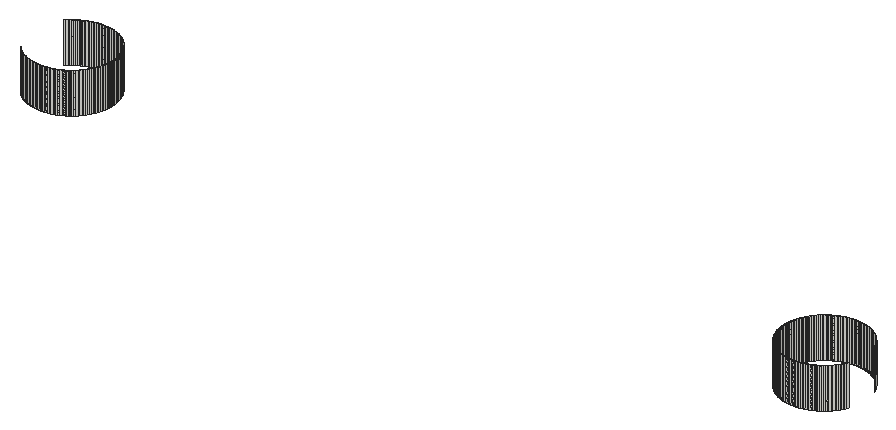
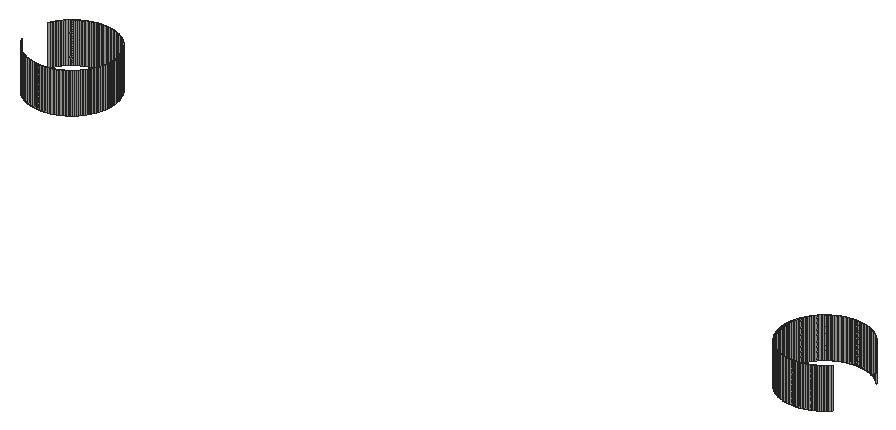
# SketchUp Ruby script. Lengths in inches.
U = 1.inch
M = Sketchup.active_model
def pt(a) = Geom::Point3d.new(a.map { |v| v * U })
def face(e, loops, mat)
  f = e.add_face(loops[0].map { |a| pt(a) })
  loops[1..].each { |l| e.add_face(l.map { |a| pt(a) }).erase! }
  f.material = f.back_material = mat if mat
  f
end
# faces: each face lists its corners as indices into pts; further lists are holes
def faces(e, pts, list, mat = nil) = list.each { |f| face(e, (f[0].is_a?(Array) ? f : [f]).map { |l| l.map { |i| pts[i] } }, mat) }
# xy, xz, yz: faces in a plane at the given z, y or x. An outline is a flat list of corners, or four numbers for a rectangle; further outlines are holes
def ring(l) = l.size == 4 ? [[l[0], l[1]], [l[2], l[1]], [l[2], l[3]], [l[0], l[3]]] : l.each_slice(2).to_a
def flat(e, list, mat, &to3) = list.each { |f| face(e, (f[0].is_a?(Array) ? f : [f]).map { |l| ring(l).map { |u, v| to3.(u, v) } }, mat) }
def xy(e, z, list, mat = nil) = flat(e, list, mat) { |x, y| [x, y, z] }
def xz(e, y, list, mat = nil) = flat(e, list, mat) { |x, z| [x, y, z] }
def yz(e, x, list, mat = nil) = flat(e, list, mat) { |y, z| [x, y, z] }
def lines(e, pts, list) = list.each { |a, b| e.add_line(pt(pts[a]), pt(pts[b])) }
# prism: a flat outline (further loops are holes) pulled along v
def prism(e, loops, v, mat = nil)
  f = face(e, loops, mat); d = Geom::Vector3d.new(v.map { |x| x * U })
  f.pushpull(f.normal.samedirection?(d) ? d.length : -d.length)
end
def box(e, o, s, mat = nil) = prism(e, [[o, [o[0] + s[0], o[1], o[2]], [o[0] + s[0], o[1] + s[1], o[2]], [o[0], o[1] + s[1], o[2]]]], [0, 0, s[2]], mat)
def at(x, y, z, deg = 0) = Geom::Transformation.translation(pt([x, y, z])) * Geom::Transformation.rotation(ORIGIN, Z_AXIS, deg.degrees)
def axes(o, x, y, z) = Geom::Transformation.new([*x, 0, *y, 0, *z, 0, *pt(o).to_a, 1])
def part(name) = M.definitions.add(name)
# library, detail: a bought-in or finely detailed component or shape, given as its bounding box
def library(name, o, s) = part(name).tap { |d| box(d.entities, o, s) }
def detail(e, o, s) = box(e.add_group.entities, o, s)
def put(e, d, t, mat = nil) = e.add_instance(d, t).tap { |i| i.material = mat if mat }
def group(e, t, mat = nil) = e.add_group.tap { |g| g.transformation = t; g.material = mat if mat }.entities
root = M.entities
xz(root,254,[[296.84,228,296.92,231],[296.92,228,297,231],[297,228,297.08,231],[297.08,228,297.16,231],[352.84,228,352.92,231],
  [352.92,228,353,231],[353,228,353.08,231],[353.08,228,353.16,231]])
xz(root,260,[[296.84,228,296.92,231],[296.92,228,297,231],[297,228,297.08,231],[297.08,228,297.16,231],[352.84,228,352.92,231],
  [352.92,228,353,231],[353,228,353.08,231],[353.08,228,353.16,231]])
yz(root,300,[[256.84,228,256.92,231],[256.92,228,257,231],[257,228,257.08,231],[257.08,228,257.16,231]])
yz(root,350,[[256.84,228,256.92,231],[256.92,228,257,231],[257,228,257.08,231],[257.08,228,257.16,231]])
p = [[296.53,254.04,228],[296.45,254.05,228],[296.45,254.05,231],[296.53,254.04,231],[296.61,254.03,228],[296.61,254.03,231],
  [296.6875,254.02,228],[296.6875,254.02,231],[296.76,254.01,228],[296.76,254.01,231],[296.84,254,228],[296.84,254,231],
  [297.24,254.01,228],[297.16,254,228],[297.16,254,231],[297.24,254.01,231],[297.3125,254.02,228],[297.3125,254.02,231],
  [297.39,254.03,228],[297.39,254.03,231],[297.47,254.04,228],[297.47,254.04,231],[297.55,254.05,228],[297.55,254.05,231],
  [352.53,254.04,228],[352.45,254.05,228],[352.45,254.05,231],[352.53,254.04,231],[352.61,254.03,228],[352.61,254.03,231],
  [352.6875,254.02,228],[352.6875,254.02,231],[352.76,254.01,228],[352.76,254.01,231],[352.84,254,228],[352.84,254,231],
  [353.24,254.01,228],[353.16,254,228],[353.16,254,231],[353.24,254.01,231],[353.3125,254.02,228],[353.3125,254.02,231],
  [353.39,254.03,228],[353.39,254.03,231],[353.47,254.04,228],[353.47,254.04,231],[353.55,254.05,228],[353.55,254.05,231],
  [296.07,254.15,228],[296,254.17,228],[296,254.17,231],[296.07,254.15,231],[296.15,254.125,228],[296.15,254.125,231],
  [296.22,254.1,228],[296.22,254.1,231],[296.3,254.08,228],[296.3,254.08,231],[296.375,254.07,228],[296.375,254.07,231],
  [297.625,254.07,228],[297.625,254.07,231],[297.7,254.08,228],[297.7,254.08,231],[297.78,254.1,228],[297.78,254.1,231],
  [297.85,254.125,228],[297.85,254.125,231],[297.93,254.15,228],[297.93,254.15,231],[298,254.17,228],[298,254.17,231],
  [352.07,254.15,228],[352,254.17,228],[352,254.17,231],[352.07,254.15,231],[352.15,254.125,228],[352.15,254.125,231],
  [352.22,254.1,228],[352.22,254.1,231],[352.3,254.08,228],[352.3,254.08,231],[352.375,254.07,228],[352.375,254.07,231],
  [353.625,254.07,228],[353.625,254.07,231],[353.7,254.08,228],[353.7,254.08,231],[353.78,254.1,228],[353.78,254.1,231],
  [353.85,254.125,228],[353.85,254.125,231],[353.93,254.15,228],[353.93,254.15,231],[354,254.17,228],[354,254.17,231],
  [295.85,254.23,228],[295.78,254.26,228],[295.78,254.26,231],[295.85,254.23,231],[295.92,254.2,228],[295.92,254.2,231],
  [298.08,254.2,228],[298.08,254.2,231],[298.15,254.23,228],[298.15,254.23,231],[298.22,254.26,228],[298.22,254.26,231],
  [351.85,254.23,228],[351.78,254.26,228],[351.78,254.26,231],[351.85,254.23,231],[351.92,254.2,228],[351.92,254.2,231],
  [354.08,254.2,228],[354.08,254.2,231],[354.15,254.23,228],[354.15,254.23,231],[354.22,254.26,228],[354.22,254.26,231],
  [295.64,254.33,228],[295.57,254.36,228],[295.57,254.36,231],[295.64,254.33,231],[295.71,254.29,228],[295.71,254.29,231],
  [298.29,254.29,228],[298.29,254.29,231],[298.36,254.33,228],[298.36,254.33,231],[298.43,254.36,228],[298.43,254.36,231],
  [351.64,254.33,228],[351.57,254.36,228],[351.57,254.36,231],[351.64,254.33,231],[351.71,254.29,228],[351.71,254.29,231],
  [354.29,254.29,228],[354.29,254.29,231],[354.36,254.33,228],[354.36,254.33,231],[354.43,254.36,228],[354.43,254.36,231],
  [295.43,254.44,228],[295.37,254.48,228],[295.37,254.48,231],[295.43,254.44,231],[295.5,254.4,228],[295.5,254.4,231],
  [298.5,254.4,228],[298.5,254.4,231],[298.57,254.44,228],[298.57,254.44,231],[298.63,254.48,228],[298.63,254.48,231],
  [351.43,254.44,228],[351.37,254.48,228],[351.37,254.48,231],[351.43,254.44,231],[351.5,254.4,228],[351.5,254.4,231],
  [354.5,254.4,228],[354.5,254.4,231],[354.57,254.44,228],[354.57,254.44,231],[354.63,254.48,228],[354.63,254.48,231],
  [295.3,254.53,228],[295.24,254.57,228],[295.24,254.57,231],[295.3,254.53,231],[298.7,254.53,228],[298.7,254.53,231],
  [298.76,254.57,228],[298.76,254.57,231],[351.3,254.53,228],[351.24,254.57,228],[351.24,254.57,231],[351.3,254.53,231],
  [354.7,254.53,228],[354.7,254.53,231],[354.76,254.57,228],[354.76,254.57,231],[295.17,254.62,228],[295.11,254.67,228],
  [295.11,254.67,231],[295.17,254.62,231],[298.83,254.62,228],[298.83,254.62,231],[298.89,254.67,228],[298.89,254.67,231],
  [351.17,254.62,228],[351.11,254.67,228],[351.11,254.67,231],[351.17,254.62,231],[354.83,254.62,228],[354.83,254.62,231],
  [354.89,254.67,228],[354.89,254.67,231],[295.05,254.72,228],[294.99,254.77,228],[294.99,254.77,231],[295.05,254.72,231],
  [298.95,254.72,228],[298.95,254.72,231],[299.01,254.77,228],[299.01,254.77,231],[351.05,254.72,228],[350.99,254.77,228],
  [350.99,254.77,231],[351.05,254.72,231],[354.95,254.72,228],[354.95,254.72,231],[355.01,254.77,228],[355.01,254.77,231],
  [294.93,254.82,228],[294.88,254.88,228],[294.88,254.88,231],[294.93,254.82,231],[299.07,254.82,228],[299.07,254.82,231],
  [299.12,254.88,228],[299.12,254.88,231],[350.93,254.82,228],[350.88,254.88,228],[350.88,254.88,231],[350.93,254.82,231],
  [355.07,254.82,228],[355.07,254.82,231],[355.12,254.88,228],[355.12,254.88,231],[294.82,254.93,228],[294.77,254.99,228],
  [294.77,254.99,231],[294.82,254.93,231],[299.18,254.93,228],[299.18,254.93,231],[299.23,254.99,228],[299.23,254.99,231],
  [350.82,254.93,228],[350.77,254.99,228],[350.77,254.99,231],[350.82,254.93,231],[355.18,254.93,228],[355.18,254.93,231],
  [355.23,254.99,228],[355.23,254.99,231],[299.28,255.05,228],[299.28,255.05,231],[350.72,255.05,228],[350.72,255.05,231],
  [355.28,255.05,228],[355.28,255.05,231],[299.33,255.11,228],[299.33,255.11,231],[299.38,255.17,228],[299.38,255.17,231],
  [350.67,255.11,228],[350.62,255.17,228],[350.62,255.17,231],[350.67,255.11,231],[355.33,255.11,228],[355.33,255.11,231],
  [355.38,255.17,228],[355.38,255.17,231],[299.43,255.24,228],[299.43,255.24,231],[299.47,255.3,228],[299.47,255.3,231],
  [350.57,255.24,228],[350.53,255.3,228],[350.53,255.3,231],[350.57,255.24,231],[355.43,255.24,228],[355.43,255.24,231],
  [355.47,255.3,228],[355.47,255.3,231],[299.52,255.37,228],[299.52,255.37,231],[350.48,255.37,228],[350.48,255.37,231],
  [355.52,255.37,228],[355.52,255.37,231],[299.56,255.43,228],[299.56,255.43,231],[299.6,255.5,228],[299.6,255.5,231],
  [350.44,255.43,228],[350.4,255.5,228],[350.4,255.5,231],[350.44,255.43,231],[355.56,255.43,228],[355.56,255.43,231],
  [355.6,255.5,228],[355.6,255.5,231],[299.64,255.57,228],[299.64,255.57,231],[350.36,255.57,228],[350.36,255.57,231],
  [355.64,255.57,228],[355.64,255.57,231],[299.67,255.64,228],[299.67,255.64,231],[299.71,255.71,228],[299.71,255.71,231],
  [350.33,255.64,228],[350.29,255.71,228],[350.29,255.71,231],[350.33,255.64,231],[355.67,255.64,228],[355.67,255.64,231],
  [355.71,255.71,228],[355.71,255.71,231],[299.74,255.78,228],[299.74,255.78,231],[350.26,255.78,228],[350.26,255.78,231],
  [355.74,255.78,228],[355.74,255.78,231],[299.77,255.85,228],[299.77,255.85,231],[350.23,255.85,228],[350.23,255.85,231],
  [299.8,255.92,228],[299.8,255.92,231],[299.83,256,228],[299.83,256,231],[350.2,255.92,228],[350.17,256,228],
  [350.17,256,231],[350.2,255.92,231],[299.85,256.07,228],[299.85,256.07,231],[350.15,256.07,228],[350.15,256.07,231],
  [299.875,256.15,228],[299.875,256.15,231],[299.9,256.22,228],[299.9,256.22,231],[350.125,256.15,228],[350.1,256.22,228],
  [350.1,256.22,231],[350.125,256.15,231],[299.92,256.3,228],[299.92,256.3,231],[350.08,256.3,228],[350.08,256.3,231],
  [299.93,256.375,228],[299.93,256.375,231],[350.07,256.375,228],[350.07,256.375,231],[299.95,256.45,228],[299.95,256.45,231],
  [350.05,256.45,228],[350.05,256.45,231],[299.96,256.53,228],[299.96,256.53,231],[299.97,256.61,228],[299.97,256.61,231],
  [350.04,256.53,228],[350.03,256.61,228],[350.03,256.61,231],[350.04,256.53,231],[299.98,256.6875,228],[299.98,256.6875,231],
  [350.02,256.6875,228],[350.02,256.6875,231],[299.99,256.76,228],[299.99,256.76,231],[350.01,256.76,228],[350.01,256.76,231],
  [300,256.84,228],[300,256.84,231],[350,256.84,228],[350,256.84,231],[299.98,257.3125,228],[299.99,257.24,228],
  [299.99,257.24,231],[299.98,257.3125,231],[300,257.16,228],[300,257.16,231],[350,257.16,228],[350.01,257.24,228],
  [350.01,257.24,231],[350,257.16,231],[350.02,257.3125,228],[350.02,257.3125,231],[299.97,257.39,228],[299.97,257.39,231],
  [350.03,257.39,228],[350.03,257.39,231],[299.96,257.47,228],[299.96,257.47,231],[350.04,257.47,228],[350.04,257.47,231],
  [299.93,257.625,228],[299.95,257.55,228],[299.95,257.55,231],[299.93,257.625,231],[350.05,257.55,228],[350.05,257.55,231],
  [350.07,257.625,228],[350.07,257.625,231],[299.92,257.7,228],[299.92,257.7,231],[350.08,257.7,228],[350.08,257.7,231],
  [299.9,257.78,228],[299.9,257.78,231],[350.1,257.78,228],[350.1,257.78,231],[299.875,257.85,228],[299.875,257.85,231],
  [350.125,257.85,228],[350.125,257.85,231],[299.83,258,228],[299.85,257.93,228],[299.85,257.93,231],[299.83,258,231],
  [350.15,257.93,228],[350.15,257.93,231],[350.17,258,228],[350.17,258,231],[299.8,258.08,228],[299.8,258.08,231],
  [350.2,258.08,228],[350.2,258.08,231],[299.74,258.22,228],[299.77,258.15,228],[299.77,258.15,231],[299.74,258.22,231],
  [350.23,258.15,228],[350.23,258.15,231],[350.26,258.22,228],[350.26,258.22,231],[299.71,258.29,228],[299.71,258.29,231],
  [350.29,258.29,228],[350.29,258.29,231],[355.71,258.29,228],[355.74,258.22,228],[355.74,258.22,231],[355.71,258.29,231],
  [299.67,258.36,228],[299.67,258.36,231],[350.33,258.36,228],[350.33,258.36,231],[355.67,258.36,228],[355.67,258.36,231],
  [299.6,258.5,228],[299.64,258.43,228],[299.64,258.43,231],[299.6,258.5,231],[350.36,258.43,228],[350.36,258.43,231],
  [350.4,258.5,228],[350.4,258.5,231],[355.6,258.5,228],[355.64,258.43,228],[355.64,258.43,231],[355.6,258.5,231],
  [299.56,258.57,228],[299.56,258.57,231],[350.44,258.57,228],[350.44,258.57,231],[355.56,258.57,228],[355.56,258.57,231],
  [299.47,258.7,228],[299.52,258.63,228],[299.52,258.63,231],[299.47,258.7,231],[350.48,258.63,228],[350.48,258.63,231],
  [350.53,258.7,228],[350.53,258.7,231],[355.47,258.7,228],[355.52,258.63,228],[355.52,258.63,231],[355.47,258.7,231],
  [299.43,258.76,228],[299.43,258.76,231],[350.57,258.76,228],[350.57,258.76,231],[355.43,258.76,228],[355.43,258.76,231],
  [299.33,258.89,228],[299.38,258.83,228],[299.38,258.83,231],[299.33,258.89,231],[350.62,258.83,228],[350.62,258.83,231],
  [350.67,258.89,228],[350.67,258.89,231],[355.33,258.89,228],[355.38,258.83,228],[355.38,258.83,231],[355.33,258.89,231],
  [299.23,259.01,228],[299.28,258.95,228],[299.28,258.95,231],[299.23,259.01,231],[350.72,258.95,228],[350.72,258.95,231],
  [350.77,259.01,228],[350.77,259.01,231],[355.23,259.01,228],[355.28,258.95,228],[355.28,258.95,231],[355.23,259.01,231],
  [294.77,259.01,228],[294.82,259.07,228],[294.82,259.07,231],[294.77,259.01,231],[299.18,259.07,228],[299.18,259.07,231],
  [350.82,259.07,228],[350.82,259.07,231],[355.18,259.07,228],[355.18,259.07,231],[294.88,259.12,228],[294.88,259.12,231],
  [294.93,259.18,228],[294.93,259.18,231],[299.07,259.18,228],[299.12,259.12,228],[299.12,259.12,231],[299.07,259.18,231],
  [350.88,259.12,228],[350.88,259.12,231],[350.93,259.18,228],[350.93,259.18,231],[355.07,259.18,228],[355.12,259.12,228],
  [355.12,259.12,231],[355.07,259.18,231],[294.99,259.23,228],[294.99,259.23,231],[295.05,259.28,228],[295.05,259.28,231],
  [298.95,259.28,228],[299.01,259.23,228],[299.01,259.23,231],[298.95,259.28,231],[350.99,259.23,228],[350.99,259.23,231],
  [351.05,259.28,228],[351.05,259.28,231],[354.95,259.28,228],[355.01,259.23,228],[355.01,259.23,231],[354.95,259.28,231],
  [295.11,259.33,228],[295.11,259.33,231],[295.17,259.38,228],[295.17,259.38,231],[298.83,259.38,228],[298.89,259.33,228],
  [298.89,259.33,231],[298.83,259.38,231],[351.11,259.33,228],[351.11,259.33,231],[351.17,259.38,228],[351.17,259.38,231],
  [354.83,259.38,228],[354.89,259.33,228],[354.89,259.33,231],[354.83,259.38,231],[295.24,259.43,228],[295.24,259.43,231],
  [295.3,259.47,228],[295.3,259.47,231],[298.7,259.47,228],[298.76,259.43,228],[298.76,259.43,231],[298.7,259.47,231],
  [351.24,259.43,228],[351.24,259.43,231],[351.3,259.47,228],[351.3,259.47,231],[354.7,259.47,228],[354.76,259.43,228],
  [354.76,259.43,231],[354.7,259.47,231],[295.37,259.52,228],[295.37,259.52,231],[295.43,259.56,228],[295.43,259.56,231],
  [298.57,259.56,228],[298.63,259.52,228],[298.63,259.52,231],[298.57,259.56,231],[351.37,259.52,228],[351.37,259.52,231],
  [351.43,259.56,228],[351.43,259.56,231],[354.57,259.56,228],[354.63,259.52,228],[354.63,259.52,231],[354.57,259.56,231],
  [295.5,259.6,228],[295.5,259.6,231],[295.57,259.64,228],[295.57,259.64,231],[295.64,259.67,228],[295.64,259.67,231],
  [298.36,259.67,228],[298.43,259.64,228],[298.43,259.64,231],[298.36,259.67,231],[298.5,259.6,228],[298.5,259.6,231],
  [351.5,259.6,228],[351.5,259.6,231],[351.57,259.64,228],[351.57,259.64,231],[351.64,259.67,228],[351.64,259.67,231],
  [354.36,259.67,228],[354.43,259.64,228],[354.43,259.64,231],[354.36,259.67,231],[354.5,259.6,228],[354.5,259.6,231],
  [295.71,259.71,228],[295.71,259.71,231],[295.78,259.74,228],[295.78,259.74,231],[295.85,259.77,228],[295.85,259.77,231],
  [298.15,259.77,228],[298.22,259.74,228],[298.22,259.74,231],[298.15,259.77,231],[298.29,259.71,228],[298.29,259.71,231],
  [351.71,259.71,228],[351.71,259.71,231],[351.78,259.74,228],[351.78,259.74,231],[351.85,259.77,228],[351.85,259.77,231],
  [354.15,259.77,228],[354.22,259.74,228],[354.22,259.74,231],[354.15,259.77,231],[354.29,259.71,228],[354.29,259.71,231],
  [295.92,259.8,228],[295.92,259.8,231],[296,259.83,228],[296,259.83,231],[296.07,259.85,228],[296.07,259.85,231],
  [297.93,259.85,228],[298,259.83,228],[298,259.83,231],[297.93,259.85,231],[298.08,259.8,228],[298.08,259.8,231],
  [351.92,259.8,228],[351.92,259.8,231],[352,259.83,228],[352,259.83,231],[352.07,259.85,228],[352.07,259.85,231],
  [353.93,259.85,228],[354,259.83,228],[354,259.83,231],[353.93,259.85,231],[354.08,259.8,228],[354.08,259.8,231],
  [296.15,259.875,228],[296.15,259.875,231],[296.22,259.9,228],[296.22,259.9,231],[296.3,259.92,228],[296.3,259.92,231],
  [296.375,259.93,228],[296.375,259.93,231],[296.45,259.95,228],[296.45,259.95,231],[296.53,259.96,228],[296.53,259.96,231],
  [297.47,259.96,228],[297.55,259.95,228],[297.55,259.95,231],[297.47,259.96,231],[297.625,259.93,228],[297.625,259.93,231],
  [297.7,259.92,228],[297.7,259.92,231],[297.78,259.9,228],[297.78,259.9,231],[297.85,259.875,228],[297.85,259.875,231],
  [352.15,259.875,228],[352.15,259.875,231],[352.22,259.9,228],[352.22,259.9,231],[352.3,259.92,228],[352.3,259.92,231],
  [352.375,259.93,228],[352.375,259.93,231],[352.45,259.95,228],[352.45,259.95,231],[352.53,259.96,228],[352.53,259.96,231],
  [353.47,259.96,228],[353.55,259.95,228],[353.55,259.95,231],[353.47,259.96,231],[353.625,259.93,228],[353.625,259.93,231],
  [353.7,259.92,228],[353.7,259.92,231],[353.78,259.9,228],[353.78,259.9,231],[353.85,259.875,228],[353.85,259.875,231],
  [296.61,259.97,228],[296.61,259.97,231],[296.6875,259.98,228],[296.6875,259.98,231],[296.76,259.99,228],[296.76,259.99,231],
  [296.84,260,228],[296.84,260,231],[297.16,260,228],[297.24,259.99,228],[297.24,259.99,231],[297.16,260,231],
  [297.3125,259.98,228],[297.3125,259.98,231],[297.39,259.97,228],[297.39,259.97,231],[352.61,259.97,228],[352.61,259.97,231],
  [352.6875,259.98,228],[352.6875,259.98,231],[352.76,259.99,228],[352.76,259.99,231],[352.84,260,228],[352.84,260,231],
  [353.16,260,228],[353.24,259.99,228],[353.24,259.99,231],[353.16,260,231],[353.3125,259.98,228],[353.3125,259.98,231],
  [353.39,259.97,228],[353.39,259.97,231]]
faces(root,p,[[0,1,2,3],[4,0,3,5],[6,4,5,7],[8,6,7,9],[10,8,9,11],[12,13,14,15],[16,12,15,17],[18,16,17,19],
  [20,18,19,21],[22,20,21,23],[24,25,26,27],[28,24,27,29],[30,28,29,31],[32,30,31,33],[34,32,33,35],[36,37,38,39],
  [40,36,39,41],[42,40,41,43],[44,42,43,45],[46,44,45,47],[48,49,50,51],[52,48,51,53],[54,52,53,55],[56,54,55,57],
  [58,56,57,59],[1,58,59,2],[60,22,23,61],[62,60,61,63],[64,62,63,65],[66,64,65,67],[68,66,67,69],[70,68,69,71],
  [72,73,74,75],[76,72,75,77],[78,76,77,79],[80,78,79,81],[82,80,81,83],[25,82,83,26],[84,46,47,85],[86,84,85,87],
  [88,86,87,89],[90,88,89,91],[92,90,91,93],[94,92,93,95],[96,97,98,99],[100,96,99,101],[49,100,101,50],[102,70,71,103],
  [104,102,103,105],[106,104,105,107],[108,109,110,111],[112,108,111,113],[73,112,113,74],[114,94,95,115],[116,114,115,117],[118,116,117,119],
  [120,121,122,123],[124,120,123,125],[97,124,125,98],[126,106,107,127],[128,126,127,129],[130,128,129,131],[132,133,134,135],[136,132,135,137],
  [109,136,137,110],[138,118,119,139],[140,138,139,141],[142,140,141,143],[144,145,146,147],[148,144,147,149],[121,148,149,122],[150,130,131,151],
  [152,150,151,153],[154,152,153,155],[156,157,158,159],[160,156,159,161],[133,160,161,134],[162,142,143,163],[164,162,163,165],[166,164,165,167],
  [168,169,170,171],[145,168,171,146],[172,154,155,173],[174,172,173,175],[176,177,178,179],[157,176,179,158],[180,166,167,181],[182,180,181,183],
  [184,185,186,187],[169,184,187,170],[188,174,175,189],[190,188,189,191],[192,193,194,195],[177,192,195,178],[196,182,183,197],[198,196,197,199],
  [200,201,202,203],[185,200,203,186],[204,190,191,205],[206,204,205,207],[208,209,210,211],[193,208,211,194],[212,198,199,213],[214,212,213,215],
  [216,217,218,219],[201,216,219,202],[220,206,207,221],[222,220,221,223],[224,225,226,227],[209,224,227,210],[228,214,215,229],[230,228,229,231],
  [232,233,234,235],[217,232,235,218],[236,222,223,237],[238,236,237,239],[240,241,242,243],[225,240,243,226],[244,230,231,245],[246,244,245,247],
  [248,238,239,249],[241,250,251,242],[252,246,247,253],[254,248,249,255],[256,254,255,257],[258,259,260,261],[250,258,261,251],[262,252,253,263],
  [264,262,263,265],[266,256,257,267],[268,266,267,269],[270,271,272,273],[259,270,273,260],[274,264,265,275],[276,274,275,277],[278,268,269,279],
  [271,280,281,272],[282,276,277,283],[284,278,279,285],[286,284,285,287],[288,289,290,291],[280,288,291,281],[292,282,283,293],[294,292,293,295],
  [296,286,287,297],[289,298,299,290],[300,294,295,301],[302,296,297,303],[304,302,303,305],[306,307,308,309],[298,306,309,299],[310,300,301,311],
  [312,310,311,313],[314,304,305,315],[307,316,317,308],[318,312,313,319],[320,314,315,321],[316,322,323,317],[324,320,321,325],[326,324,325,327],
  [328,329,330,331],[322,328,331,323],[332,326,327,333],[329,334,335,330],[336,332,333,337],[338,336,337,339],[340,341,342,343],[334,340,343,335],
  [344,338,339,345],[341,346,347,342],[348,344,345,349],[346,350,351,347],[352,348,349,353],[350,354,355,351],[356,352,353,357],[358,356,357,359],
  [360,361,362,363],[354,360,363,355],[364,358,359,365],[361,366,367,362],[368,364,365,369],[366,370,371,367],[372,368,369,373],[370,374,375,371],
  [376,377,378,379],[377,380,381,378],[382,383,384,385],[383,386,387,384],[388,376,379,389],[386,390,391,387],[392,388,389,393],[390,394,395,391],
  [396,397,398,399],[397,392,393,398],[394,400,401,395],[400,402,403,401],[404,396,399,405],[402,406,407,403],[408,404,405,409],[406,410,411,407],
  [412,408,409,413],[410,414,415,411],[416,417,418,419],[417,412,413,418],[414,420,421,415],[420,422,423,421],[424,416,419,425],[422,426,427,423],
  [428,429,430,431],[429,424,425,430],[426,432,433,427],[432,434,435,433],[436,428,431,437],[434,438,439,435],[440,441,442,443],[444,436,437,445],
  [438,446,447,439],[448,440,443,449],[450,451,452,453],[451,444,445,452],[446,454,455,447],[454,456,457,455],[458,459,460,461],[459,448,449,460],
  [462,450,453,463],[456,464,465,457],[466,458,461,467],[468,469,470,471],[469,462,463,470],[464,472,473,465],[472,474,475,473],[476,477,478,479],
  [477,466,467,478],[480,468,471,481],[474,482,483,475],[484,476,479,485],[486,487,488,489],[487,480,481,488],[482,490,491,483],[490,492,493,491],
  [494,495,496,497],[495,484,485,496],[498,499,500,501],[499,486,489,500],[492,502,503,493],[502,504,505,503],[506,507,508,509],[507,494,497,508],
  [510,511,512,513],[514,498,501,515],[504,516,517,505],[518,506,509,519],[511,520,521,512],[520,522,523,521],[524,525,526,527],[525,514,515,526],
  [516,528,529,517],[528,530,531,529],[532,533,534,535],[533,518,519,534],[522,536,537,523],[536,538,539,537],[540,541,542,543],[541,524,527,542],
  [530,544,545,531],[544,546,547,545],[548,549,550,551],[549,532,535,550],[538,552,553,539],[552,554,555,553],[556,557,558,559],[557,540,543,558],
  [546,560,561,547],[560,562,563,561],[564,565,566,567],[565,548,551,566],[554,568,569,555],[568,570,571,569],[572,573,574,575],[573,556,559,574],
  [562,576,577,563],[576,578,579,577],[580,581,582,583],[581,564,567,582],[570,584,585,571],[584,586,587,585],[588,589,590,591],[589,572,575,590],
  [578,592,593,579],[592,594,595,593],[596,597,598,599],[597,580,583,598],[586,600,601,587],[600,602,603,601],[602,604,605,603],[606,607,608,609],
  [607,610,611,608],[610,588,591,611],[594,612,613,595],[612,614,615,613],[614,616,617,615],[618,619,620,621],[619,622,623,620],[622,596,599,623],
  [604,624,625,605],[624,626,627,625],[626,628,629,627],[630,631,632,633],[631,634,635,632],[634,606,609,635],[616,636,637,617],[636,638,639,637],
  [638,640,641,639],[642,643,644,645],[643,646,647,644],[646,618,621,647],[628,648,649,629],[648,650,651,649],[650,652,653,651],[654,655,656,657],
  [655,658,659,656],[658,630,633,659],[640,660,661,641],[660,662,663,661],[662,664,665,663],[666,667,668,669],[667,670,671,668],[670,642,645,671],
  [652,672,673,653],[672,674,675,673],[674,676,677,675],[676,678,679,677],[678,680,681,679],[680,682,683,681],[684,685,686,687],[685,688,689,686],
  [688,690,691,689],[690,692,693,691],[692,694,695,693],[694,654,657,695],[664,696,697,665],[696,698,699,697],[698,700,701,699],[700,702,703,701],
  [702,704,705,703],[704,706,707,705],[708,709,710,711],[709,712,713,710],[712,714,715,713],[714,716,717,715],[716,718,719,717],[718,666,669,719],
  [682,720,721,683],[720,722,723,721],[722,724,725,723],[724,726,727,725],[728,729,730,731],[729,732,733,730],[732,734,735,733],[734,684,687,735],
  [706,736,737,707],[736,738,739,737],[738,740,741,739],[740,742,743,741],[744,745,746,747],[745,748,749,746],[748,750,751,749],[750,708,711,751]])
